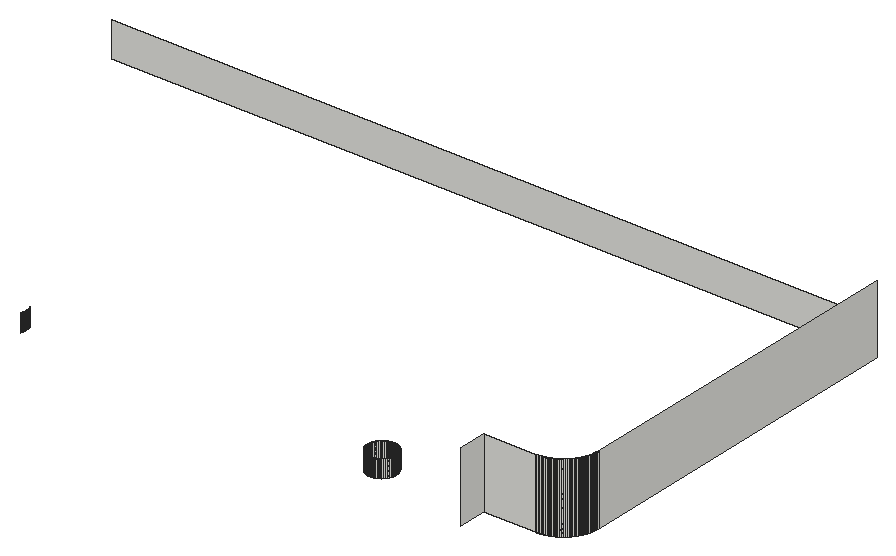
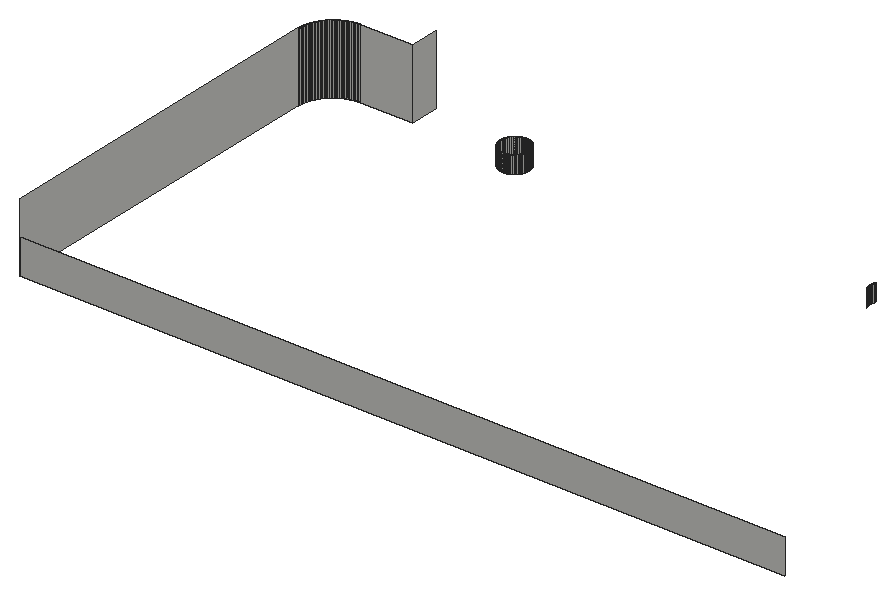
# SketchUp Ruby script. Lengths in inches.
U = 1.inch
M = Sketchup.active_model
def pt(a) = Geom::Point3d.new(a.map { |v| v * U })
def face(e, loops, mat)
  f = e.add_face(loops[0].map { |a| pt(a) })
  loops[1..].each { |l| e.add_face(l.map { |a| pt(a) }).erase! }
  f.material = f.back_material = mat if mat
  f
end
# faces: each face lists its corners as indices into pts; further lists are holes
def faces(e, pts, list, mat = nil) = list.each { |f| face(e, (f[0].is_a?(Array) ? f : [f]).map { |l| l.map { |i| pts[i] } }, mat) }
# xy, xz, yz: faces in a plane at the given z, y or x. An outline is a flat list of corners, or four numbers for a rectangle; further outlines are holes
def ring(l) = l.size == 4 ? [[l[0], l[1]], [l[2], l[1]], [l[2], l[3]], [l[0], l[3]]] : l.each_slice(2).to_a
def flat(e, list, mat, &to3) = list.each { |f| face(e, (f[0].is_a?(Array) ? f : [f]).map { |l| ring(l).map { |u, v| to3.(u, v) } }, mat) }
def xy(e, z, list, mat = nil) = flat(e, list, mat) { |x, y| [x, y, z] }
def xz(e, y, list, mat = nil) = flat(e, list, mat) { |x, z| [x, y, z] }
def yz(e, x, list, mat = nil) = flat(e, list, mat) { |y, z| [x, y, z] }
def lines(e, pts, list) = list.each { |a, b| e.add_line(pt(pts[a]), pt(pts[b])) }
# prism: a flat outline (further loops are holes) pulled along v
def prism(e, loops, v, mat = nil)
  f = face(e, loops, mat); d = Geom::Vector3d.new(v.map { |x| x * U })
  f.pushpull(f.normal.samedirection?(d) ? d.length : -d.length)
end
def box(e, o, s, mat = nil) = prism(e, [[o, [o[0] + s[0], o[1], o[2]], [o[0] + s[0], o[1] + s[1], o[2]], [o[0], o[1] + s[1], o[2]]]], [0, 0, s[2]], mat)
def at(x, y, z, deg = 0) = Geom::Transformation.translation(pt([x, y, z])) * Geom::Transformation.rotation(ORIGIN, Z_AXIS, deg.degrees)
def axes(o, x, y, z) = Geom::Transformation.new([*x, 0, *y, 0, *z, 0, *pt(o).to_a, 1])
def part(name) = M.definitions.add(name)
# library, detail: a bought-in or finely detailed component or shape, given as its bounding box
def library(name, o, s) = part(name).tap { |d| box(d.entities, o, s) }
def detail(e, o, s) = box(e.add_group.entities, o, s)
def put(e, d, t, mat = nil) = e.add_instance(d, t).tap { |i| i.material = mat if mat }
def group(e, t, mat = nil) = e.add_group.tap { |g| g.transformation = t; g.material = mat if mat }.entities
root = M.entities
xz(root,124,[[250.84,366,250.92,369],[250.92,366,251,369],[251,366,251.08,369],[251.08,366,251.16,369]])
xz(root,126,[[269,366,278,378],[278,366,278.12,378],[278.12,366,278.24,378]])
xz(root,129,[[250.84,366,250.92,369],[250.92,366,251,369],[251,366,251.08,369],[251.08,366,251.16,369]])
xz(root,192,[[152,366,284,372]])
yz(root,189.61,[[126.1875,366,126.26,369],[126.74,366,126.8125,369]])
yz(root,189.625,[[126.42,366,126.5,369],[126.5,366,126.58,369]])
yz(root,248.5,[[126.34,366,126.42,369],[126.42,366,126.5,369],[126.5,366,126.58,369],[126.58,366,126.66,369]])
yz(root,253.49,[[126.26,366,126.34,369],[126.66,366,126.74,369]])
yz(root,253.5,[[126.42,366,126.5,369],[126.5,366,126.58,369]])
yz(root,269,[[121,366,126,378]])
yz(root,284,[[131.76,366,131.88,378],[131.88,366,132,378],[132,366,192,378]])
p = [[250.53,124.04,366],[250.45,124.06,366],[250.45,124.06,369],[250.53,124.04,369],[250.61,124.03,366],[250.61,124.03,369],
  [250.6875,124.02,366],[250.6875,124.02,369],[250.76,124.01,366],[250.76,124.01,369],[250.84,124,366],[250.84,124,369],
  [251.24,124.01,366],[251.16,124,366],[251.16,124,369],[251.24,124.01,369],[251.3125,124.02,366],[251.3125,124.02,369],
  [251.39,124.03,366],[251.39,124.03,369],[251.47,124.04,366],[251.47,124.04,369],[251.55,124.06,366],[251.55,124.06,369],
  [250.15,124.15,366],[250.08,124.18,366],[250.08,124.18,369],[250.15,124.15,369],[250.23,124.12,366],[250.23,124.12,369],
  [250.3,124.1,366],[250.3,124.1,369],[250.38,124.08,366],[250.38,124.08,369],[251.62,124.08,366],[251.62,124.08,369],
  [251.7,124.1,366],[251.7,124.1,369],[251.77,124.12,366],[251.77,124.12,369],[251.85,124.15,366],[251.85,124.15,369],
  [251.92,124.18,366],[251.92,124.18,369],[249.94,124.24,366],[249.86,124.27,366],[249.86,124.27,369],[249.94,124.24,369],
  [250.01,124.21,366],[250.01,124.21,369],[251.99,124.21,366],[251.99,124.21,369],[252.0625,124.24,366],[252.0625,124.24,369],
  [252.13,124.27,366],[252.13,124.27,369],[249.73,124.35,366],[249.66,124.39,366],[249.66,124.39,369],[249.73,124.35,369],
  [249.8,124.31,366],[249.8,124.31,369],[252.2,124.31,366],[252.2,124.31,369],[252.27,124.35,366],[252.27,124.35,369],
  [252.34,124.39,366],[252.34,124.39,369],[249.59,124.43,366],[249.53,124.48,366],[249.53,124.48,369],[249.59,124.43,369],
  [252.41,124.43,366],[252.41,124.43,369],[252.47,124.48,366],[252.47,124.48,369],[249.47,124.52,366],[249.41,124.57,366],
  [249.41,124.57,369],[249.47,124.52,369],[252.53,124.52,366],[252.53,124.52,369],[252.59,124.57,366],[252.59,124.57,369],
  [249.35,124.625,366],[249.29,124.68,366],[249.29,124.68,369],[249.35,124.625,369],[252.65,124.625,366],[252.65,124.625,369],
  [252.71,124.68,366],[252.71,124.68,369],[249.23,124.73,366],[249.18,124.79,366],[249.18,124.79,369],[249.23,124.73,369],
  [252.77,124.73,366],[252.77,124.73,369],[252.82,124.79,366],[252.82,124.79,369],[249.125,124.85,366],[249.07,124.91,366],
  [249.07,124.91,369],[249.125,124.85,369],[252.875,124.85,366],[252.875,124.85,369],[252.93,124.91,366],[252.93,124.91,369],
  [249.02,124.97,366],[249.02,124.97,369],[252.98,124.97,366],[252.98,124.97,369],[248.98,125.03,366],[248.93,125.09,366],
  [248.93,125.09,369],[248.98,125.03,369],[253.02,125.03,366],[253.02,125.03,369],[253.07,125.09,366],[253.07,125.09,369],
  [248.89,125.16,366],[248.89,125.16,369],[253.11,125.16,366],[253.11,125.16,369],[248.85,125.23,366],[248.81,125.3,366],
  [248.81,125.3,369],[248.85,125.23,369],[253.15,125.23,366],[253.15,125.23,369],[253.19,125.3,366],[253.19,125.3,369],
  [248.77,125.37,366],[248.77,125.37,369],[253.23,125.37,366],[253.23,125.37,369],[189.42,125.51,366],[189.39,125.4375,366],
  [189.39,125.4375,369],[189.42,125.51,369],[248.74,125.4375,366],[248.71,125.51,366],[248.71,125.51,369],[248.74,125.4375,369],
  [253.26,125.4375,366],[253.26,125.4375,369],[253.29,125.51,366],[253.29,125.51,369],[189.45,125.58,366],[189.45,125.58,369],
  [248.68,125.58,366],[248.68,125.58,369],[253.32,125.58,366],[253.32,125.58,369],[189.48,125.65,366],[189.48,125.65,369],
  [248.65,125.65,366],[248.65,125.65,369],[253.35,125.65,366],[253.35,125.65,369],[189.5,125.73,366],[189.5,125.73,369],
  [189.53,125.8,366],[189.53,125.8,369],[248.62,125.73,366],[248.6,125.8,366],[248.6,125.8,369],[248.62,125.73,369],
  [253.38,125.73,366],[253.38,125.73,369],[253.4,125.8,366],[253.4,125.8,369],[189.55,125.88,366],[189.55,125.88,369],
  [248.58,125.88,366],[248.58,125.88,369],[253.42,125.88,366],[253.42,125.88,369],[189.56,125.95,366],[189.56,125.95,369],
  [248.56,125.95,366],[248.56,125.95,369],[253.44,125.95,366],[253.44,125.95,369],[189.58,126.03,366],[189.58,126.03,369],
  [189.59,126.11,366],[189.59,126.11,369],[248.54,126.03,366],[248.53,126.11,366],[248.53,126.11,369],[248.54,126.03,369],
  [253.46,126.03,366],[253.46,126.03,369],[253.47,126.11,366],[253.47,126.11,369],[278.35,126.01,378],[278.24,126,378],
  [278.24,126,366],[278.35,126.01,366],[278.47,126.02,378],[278.47,126.02,366],[278.59,126.03,378],[278.59,126.03,366],
  [278.71,126.04,378],[278.71,126.04,366],[278.82,126.06,378],[278.82,126.06,366],[189.61,126.1875,366],[189.61,126.1875,369],
  [248.52,126.1875,366],[248.52,126.1875,369],[253.48,126.1875,366],[253.48,126.1875,369],[278.9375,126.07,378],[278.9375,126.07,366],
  [279.05,126.09,378],[279.05,126.09,366],[279.17,126.12,378],[279.17,126.12,366],[279.29,126.14,378],[279.29,126.14,366],
  [279.4,126.17,378],[279.4,126.17,366],[248.51,126.26,366],[248.51,126.26,369],[253.49,126.26,366],[253.49,126.26,369],
  [279.51,126.19,378],[279.51,126.19,366],[279.63,126.23,378],[279.63,126.23,366],[279.74,126.26,378],[279.74,126.26,366],
  [189.62,126.34,366],[189.61,126.26,366],[189.61,126.26,369],[189.62,126.34,369],[189.625,126.42,366],[189.625,126.42,369],
  [248.5,126.34,366],[248.5,126.34,369],[253.5,126.42,366],[253.49,126.34,366],[253.49,126.34,369],[253.5,126.42,369],
  [279.85,126.29,378],[279.85,126.29,366],[279.97,126.33,378],[279.97,126.33,366],[280.08,126.37,378],[280.08,126.37,366],
  [280.1875,126.41,378],[280.1875,126.41,366],[280.3,126.46,378],[280.3,126.46,366],[280.4,126.5,378],[280.4,126.5,366],
  [280.51,126.55,378],[280.51,126.55,366],[189.62,126.66,366],[189.625,126.58,366],[189.625,126.58,369],[189.62,126.66,369],
  [253.49,126.66,366],[253.5,126.58,366],[253.5,126.58,369],[253.49,126.66,369],[280.62,126.6,378],[280.62,126.6,366],
  [280.72,126.65,378],[280.72,126.65,366],[189.61,126.74,366],[189.61,126.74,369],[248.5,126.66,366],[248.51,126.74,366],
  [248.51,126.74,369],[248.5,126.66,369],[248.52,126.8125,366],[248.52,126.8125,369],[253.48,126.8125,366],[253.49,126.74,366],
  [253.49,126.74,369],[253.48,126.8125,369],[280.83,126.71,378],[280.83,126.71,366],[280.93,126.77,378],[280.93,126.77,366],
  [189.59,126.89,366],[189.61,126.8125,366],[189.61,126.8125,369],[189.59,126.89,369],[248.53,126.89,366],[248.53,126.89,369],
  [253.47,126.89,366],[253.47,126.89,369],[281.03,126.82,378],[281.03,126.82,366],[281.13,126.88,378],[281.13,126.88,366],
  [189.58,126.97,366],[189.58,126.97,369],[248.54,126.97,366],[248.54,126.97,369],[253.46,126.97,366],[253.46,126.97,369],
  [281.23,126.95,378],[281.23,126.95,366],[281.33,127.01,378],[281.33,127.01,366],[189.55,127.12,366],[189.56,127.05,366],
  [189.56,127.05,369],[189.55,127.12,369],[248.56,127.05,366],[248.56,127.05,369],[248.58,127.12,366],[248.58,127.12,369],
  [253.42,127.12,366],[253.44,127.05,366],[253.44,127.05,369],[253.42,127.12,369],[281.43,127.08,378],[281.43,127.08,366],
  [189.53,127.2,366],[189.53,127.2,369],[248.6,127.2,366],[248.6,127.2,369],[253.4,127.2,366],[253.4,127.2,369],
  [281.53,127.15,378],[281.53,127.15,366],[281.62,127.22,378],[281.62,127.22,366],[189.5,127.27,366],[189.5,127.27,369],
  [248.62,127.27,366],[248.62,127.27,369],[253.38,127.27,366],[253.38,127.27,369],[281.71,127.29,378],[281.71,127.29,366],
  [189.45,127.42,366],[189.48,127.35,366],[189.48,127.35,369],[189.45,127.42,369],[248.65,127.35,366],[248.65,127.35,369],
  [248.68,127.42,366],[248.68,127.42,369],[253.32,127.42,366],[253.35,127.35,366],[253.35,127.35,369],[253.32,127.42,369],
  [281.81,127.36,378],[281.81,127.36,366],[189.42,127.49,366],[189.42,127.49,369],[248.71,127.49,366],[248.71,127.49,369],
  [253.29,127.49,366],[253.29,127.49,369],[281.9,127.4375,378],[281.9,127.4375,366],[281.99,127.51,378],[281.99,127.51,366],
  [189.39,127.5625,366],[189.39,127.5625,369],[248.74,127.5625,366],[248.74,127.5625,369],[253.26,127.5625,366],[253.26,127.5625,369],
  [282.07,127.59,378],[282.07,127.59,366],[189.35,127.63,366],[189.35,127.63,369],[248.77,127.63,366],[248.77,127.63,369],
  [248.81,127.7,366],[248.81,127.7,369],[253.19,127.7,366],[253.23,127.63,366],[253.23,127.63,369],[253.19,127.7,369],
  [282.16,127.67,378],[282.16,127.67,366],[248.85,127.77,366],[248.85,127.77,369],[253.15,127.77,366],[253.15,127.77,369],
  [282.24,127.76,378],[282.24,127.76,366],[248.89,127.84,366],[248.89,127.84,369],[248.93,127.91,366],[248.93,127.91,369],
  [253.07,127.91,366],[253.11,127.84,366],[253.11,127.84,369],[253.07,127.91,369],[282.33,127.84,378],[282.33,127.84,366],
  [282.41,127.93,378],[282.41,127.93,366],[248.98,127.97,366],[248.98,127.97,369],[253.02,127.97,366],[253.02,127.97,369],
  [282.48,128.01,378],[282.48,128.01,366],[249.02,128.03,366],[249.02,128.03,369],[249.07,128.09,366],[249.07,128.09,369],
  [252.93,128.09,366],[252.98,128.03,366],[252.98,128.03,369],[252.93,128.09,369],[282.5625,128.1,378],[282.5625,128.1,366],
  [249.125,128.15,366],[249.125,128.15,369],[252.875,128.15,366],[252.875,128.15,369],[282.64,128.19,378],[282.64,128.19,366],
  [249.18,128.21,366],[249.18,128.21,369],[249.23,128.27,366],[249.23,128.27,369],[252.77,128.27,366],[252.82,128.21,366],
  [252.82,128.21,369],[252.77,128.27,369],[282.71,128.29,378],[282.71,128.29,366],[249.29,128.32,366],[249.29,128.32,369],
  [249.35,128.375,366],[249.35,128.375,369],[252.65,128.375,366],[252.71,128.32,366],[252.71,128.32,369],[252.65,128.375,369],
  [282.78,128.38,378],[282.78,128.38,366],[249.41,128.43,366],[249.41,128.43,369],[249.47,128.48,366],[249.47,128.48,369],
  [252.53,128.48,366],[252.59,128.43,366],[252.59,128.43,369],[252.53,128.48,369],[282.85,128.47,378],[282.85,128.47,366],
  [249.53,128.52,366],[249.53,128.52,369],[249.59,128.57,366],[249.59,128.57,369],[252.41,128.57,366],[252.47,128.52,366],
  [252.47,128.52,369],[252.41,128.57,369],[282.92,128.57,378],[282.92,128.57,366],[249.66,128.61,366],[249.66,128.61,369],
  [249.73,128.65,366],[249.73,128.65,369],[252.27,128.65,366],[252.34,128.61,366],[252.34,128.61,369],[252.27,128.65,369],
  [282.99,128.67,378],[282.99,128.67,366],[249.8,128.69,366],[249.8,128.69,369],[249.86,128.73,366],[249.86,128.73,369],
  [249.94,128.76,366],[249.94,128.76,369],[252.0625,128.76,366],[252.13,128.73,366],[252.13,128.73,369],[252.0625,128.76,369],
  [252.2,128.69,366],[252.2,128.69,369],[283.05,128.77,378],[283.05,128.77,366],[250.01,128.79,366],[250.01,128.79,369],
  [250.08,128.82,366],[250.08,128.82,369],[250.15,128.85,366],[250.15,128.85,369],[251.85,128.85,366],[251.92,128.82,366],
  [251.92,128.82,369],[251.85,128.85,369],[251.99,128.79,366],[251.99,128.79,369],[283.12,128.87,378],[283.12,128.87,366],
  [250.23,128.88,366],[250.23,128.88,369],[250.3,128.9,366],[250.3,128.9,369],[250.38,128.92,366],[250.38,128.92,369],
  [250.45,128.94,366],[250.45,128.94,369],[250.53,128.96,366],[250.53,128.96,369],[251.47,128.96,366],[251.55,128.94,366],
  [251.55,128.94,369],[251.47,128.96,369],[251.62,128.92,366],[251.62,128.92,369],[251.7,128.9,366],[251.7,128.9,369],
  [251.77,128.88,366],[251.77,128.88,369],[283.18,128.97,378],[283.18,128.97,366],[250.61,128.97,366],[250.61,128.97,369],
  [250.6875,128.98,366],[250.6875,128.98,369],[250.76,128.99,366],[250.76,128.99,369],[250.84,129,366],[250.84,129,369],
  [251.16,129,366],[251.24,128.99,366],[251.24,128.99,369],[251.16,129,369],[251.3125,128.98,366],[251.3125,128.98,369],
  [251.39,128.97,366],[251.39,128.97,369],[283.23,129.07,378],[283.23,129.07,366],[283.29,129.17,378],[283.29,129.17,366],
  [283.35,129.28,378],[283.35,129.28,366],[283.4,129.38,378],[283.4,129.38,366],[283.45,129.49,378],[283.45,129.49,366],
  [283.5,129.6,378],[283.5,129.6,366],[283.54,129.7,378],[283.54,129.7,366],[283.59,129.8125,378],[283.59,129.8125,366],
  [283.63,129.92,378],[283.63,129.92,366],[283.67,130.03,378],[283.67,130.03,366],[283.71,130.15,378],[283.71,130.15,366],
  [283.74,130.26,378],[283.74,130.26,366],[283.77,130.37,378],[283.77,130.37,366],[283.81,130.49,378],[283.81,130.49,366],
  [283.83,130.6,378],[283.83,130.6,366],[283.86,130.71,378],[283.86,130.71,366],[283.88,130.83,378],[283.88,130.83,366],
  [283.91,130.95,378],[283.91,130.95,366],[283.93,131.0625,378],[283.93,131.0625,366],[283.94,131.18,378],[283.94,131.18,366],
  [283.96,131.29,378],[283.96,131.29,366],[283.97,131.41,378],[283.97,131.41,366],[283.98,131.53,378],[283.98,131.53,366],
  [283.99,131.65,378],[283.99,131.65,366],[284,131.76,378],[284,131.76,366]]
faces(root,p,[[0,1,2,3],[4,0,3,5],[6,4,5,7],[8,6,7,9],[10,8,9,11],[12,13,14,15],[16,12,15,17],[18,16,17,19],
  [20,18,19,21],[22,20,21,23],[24,25,26,27],[28,24,27,29],[30,28,29,31],[32,30,31,33],[1,32,33,2],[34,22,23,35],
  [36,34,35,37],[38,36,37,39],[40,38,39,41],[42,40,41,43],[44,45,46,47],[48,44,47,49],[25,48,49,26],[50,42,43,51],
  [52,50,51,53],[54,52,53,55],[56,57,58,59],[60,56,59,61],[45,60,61,46],[62,54,55,63],[64,62,63,65],[66,64,65,67],
  [68,69,70,71],[57,68,71,58],[72,66,67,73],[74,72,73,75],[76,77,78,79],[69,76,79,70],[80,74,75,81],[82,80,81,83],
  [84,85,86,87],[77,84,87,78],[88,82,83,89],[90,88,89,91],[92,93,94,95],[85,92,95,86],[96,90,91,97],[98,96,97,99],
  [100,101,102,103],[93,100,103,94],[104,98,99,105],[106,104,105,107],[101,108,109,102],[110,106,107,111],[112,113,114,115],[108,112,115,109],
  [116,110,111,117],[118,116,117,119],[113,120,121,114],[122,118,119,123],[124,125,126,127],[120,124,127,121],[128,122,123,129],[130,128,129,131],
  [125,132,133,126],[134,130,131,135],[136,137,138,139],[140,141,142,143],[132,140,143,133],[144,134,135,145],[146,144,145,147],[148,136,139,149],
  [141,150,151,142],[152,146,147,153],[154,148,149,155],[150,156,157,151],[158,152,153,159],[160,154,155,161],[162,160,161,163],[164,165,166,167],
  [156,164,167,157],[168,158,159,169],[170,168,169,171],[172,162,163,173],[165,174,175,166],[176,170,171,177],[178,172,173,179],[174,180,181,175],
  [182,176,177,183],[184,178,179,185],[186,184,185,187],[188,189,190,191],[180,188,191,181],[192,182,183,193],[194,192,193,195],[196,197,198,199],
  [200,196,199,201],[202,200,201,203],[204,202,203,205],[206,204,205,207],[208,186,187,209],[189,210,211,190],[212,194,195,213],[214,206,207,215],
  [216,214,215,217],[218,216,217,219],[220,218,219,221],[222,220,221,223],[210,224,225,211],[226,212,213,227],[228,222,223,229],[230,228,229,231],
  [232,230,231,233],[234,235,236,237],[238,234,237,239],[224,240,241,225],[242,243,244,245],[246,232,233,247],[248,246,247,249],[250,248,249,251],
  [252,250,251,253],[254,252,253,255],[256,254,255,257],[258,256,257,259],[260,261,262,263],[264,265,266,267],[268,258,259,269],[270,268,269,271],
  [272,260,263,273],[274,275,276,277],[275,278,279,276],[280,281,282,283],[284,270,271,285],[286,284,285,287],[288,289,290,291],[278,292,293,279],
  [294,280,283,295],[296,286,287,297],[298,296,297,299],[300,288,291,301],[292,302,303,293],[304,294,295,305],[306,298,299,307],[308,306,307,309],
  [310,311,312,313],[311,300,301,312],[302,314,315,303],[314,316,317,315],[318,319,320,321],[319,304,305,320],[322,308,309,323],[324,310,313,325],
  [316,326,327,317],[328,318,321,329],[330,322,323,331],[332,330,331,333],[334,324,325,335],[326,336,337,327],[338,328,329,339],[340,332,333,341],
  [342,343,344,345],[343,334,335,344],[336,346,347,337],[346,348,349,347],[350,351,352,353],[351,338,339,352],[354,340,341,355],[356,342,345,357],
  [348,358,359,349],[360,350,353,361],[362,354,355,363],[364,362,363,365],[366,356,357,367],[358,368,369,359],[370,360,361,371],[372,364,365,373],
  [374,366,367,375],[368,376,377,369],[376,378,379,377],[380,381,382,383],[381,370,371,382],[384,372,373,385],[378,386,387,379],[388,380,383,389],
  [390,384,385,391],[386,392,393,387],[392,394,395,393],[396,397,398,399],[397,388,389,398],[400,390,391,401],[402,400,401,403],[394,404,405,395],
  [406,396,399,407],[408,402,403,409],[404,410,411,405],[410,412,413,411],[414,415,416,417],[415,406,407,416],[418,408,409,419],[412,420,421,413],
  [422,414,417,423],[424,418,419,425],[420,426,427,421],[426,428,429,427],[430,431,432,433],[431,422,423,432],[434,424,425,435],[428,436,437,429],
  [436,438,439,437],[440,441,442,443],[441,430,433,442],[444,434,435,445],[438,446,447,439],[446,448,449,447],[450,451,452,453],[451,440,443,452],
  [454,444,445,455],[448,456,457,449],[456,458,459,457],[460,461,462,463],[461,450,453,462],[464,454,455,465],[458,466,467,459],[466,468,469,467],
  [470,471,472,473],[471,460,463,472],[474,464,465,475],[468,476,477,469],[476,478,479,477],[478,480,481,479],[482,483,484,485],[483,486,487,484],
  [486,470,473,487],[488,474,475,489],[480,490,491,481],[490,492,493,491],[492,494,495,493],[496,497,498,499],[497,500,501,498],[500,482,485,501],
  [502,488,489,503],[494,504,505,495],[504,506,507,505],[506,508,509,507],[508,510,511,509],[510,512,513,511],[514,515,516,517],[515,518,519,516],
  [518,520,521,519],[520,522,523,521],[522,496,499,523],[524,502,503,525],[512,526,527,513],[526,528,529,527],[528,530,531,529],[530,532,533,531],
  [534,535,536,537],[535,538,539,536],[538,540,541,539],[540,514,517,541],[542,524,525,543],[544,542,543,545],[546,544,545,547],[548,546,547,549],
  [550,548,549,551],[552,550,551,553],[554,552,553,555],[556,554,555,557],[558,556,557,559],[560,558,559,561],[562,560,561,563],[564,562,563,565],
  [566,564,565,567],[568,566,567,569],[570,568,569,571],[572,570,571,573],[574,572,573,575],[576,574,575,577],[578,576,577,579],[580,578,579,581],
  [582,580,581,583],[584,582,583,585],[586,584,585,587],[588,586,587,589],[590,588,589,591]])
